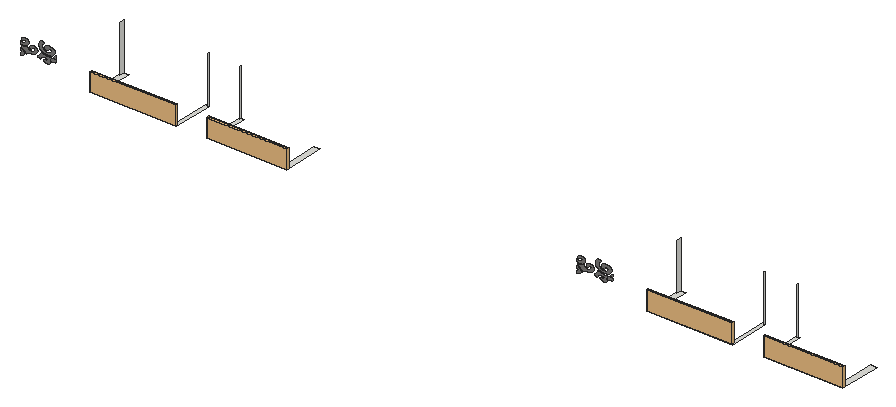
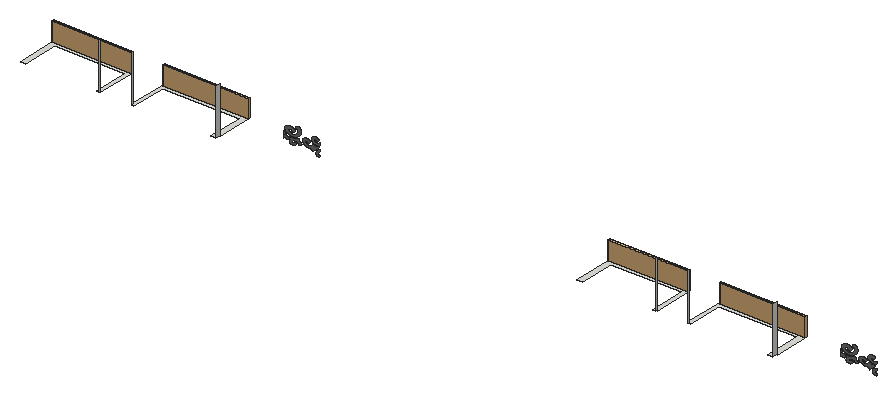
# SketchUp Ruby script. Lengths in inches.
U = 1.inch
M = Sketchup.active_model
def pt(a) = Geom::Point3d.new(a.map { |v| v * U })
def face(e, loops, mat)
  f = e.add_face(loops[0].map { |a| pt(a) })
  loops[1..].each { |l| e.add_face(l.map { |a| pt(a) }).erase! }
  f.material = f.back_material = mat if mat
  f
end
# faces: each face lists its corners as indices into pts; further lists are holes
def faces(e, pts, list, mat = nil) = list.each { |f| face(e, (f[0].is_a?(Array) ? f : [f]).map { |l| l.map { |i| pts[i] } }, mat) }
# xy, xz, yz: faces in a plane at the given z, y or x. An outline is a flat list of corners, or four numbers for a rectangle; further outlines are holes
def ring(l) = l.size == 4 ? [[l[0], l[1]], [l[2], l[1]], [l[2], l[3]], [l[0], l[3]]] : l.each_slice(2).to_a
def flat(e, list, mat, &to3) = list.each { |f| face(e, (f[0].is_a?(Array) ? f : [f]).map { |l| ring(l).map { |u, v| to3.(u, v) } }, mat) }
def xy(e, z, list, mat = nil) = flat(e, list, mat) { |x, y| [x, y, z] }
def xz(e, y, list, mat = nil) = flat(e, list, mat) { |x, z| [x, y, z] }
def yz(e, x, list, mat = nil) = flat(e, list, mat) { |y, z| [x, y, z] }
def lines(e, pts, list) = list.each { |a, b| e.add_line(pt(pts[a]), pt(pts[b])) }
# prism: a flat outline (further loops are holes) pulled along v
def prism(e, loops, v, mat = nil)
  f = face(e, loops, mat); d = Geom::Vector3d.new(v.map { |x| x * U })
  f.pushpull(f.normal.samedirection?(d) ? d.length : -d.length)
end
def box(e, o, s, mat = nil) = prism(e, [[o, [o[0] + s[0], o[1], o[2]], [o[0] + s[0], o[1] + s[1], o[2]], [o[0], o[1] + s[1], o[2]]]], [0, 0, s[2]], mat)
def at(x, y, z, deg = 0) = Geom::Transformation.translation(pt([x, y, z])) * Geom::Transformation.rotation(ORIGIN, Z_AXIS, deg.degrees)
def axes(o, x, y, z) = Geom::Transformation.new([*x, 0, *y, 0, *z, 0, *pt(o).to_a, 1])
def part(name) = M.definitions.add(name)
# library, detail: a bought-in or finely detailed component or shape, given as its bounding box
def library(name, o, s) = part(name).tap { |d| box(d.entities, o, s) }
def detail(e, o, s) = box(e.add_group.entities, o, s)
def put(e, d, t, mat = nil) = e.add_instance(d, t).tap { |i| i.material = mat if mat }
def group(e, t, mat = nil) = e.add_group.tap { |g| g.transformation = t; g.material = mat if mat }.entities
root = M.entities
M.materials.add("[0043_SaddleBrown]4").color = [124, 123, 122]
c1 = library("Glass Railing",[0,0,0],[139.5,4.76,42])
xy(root,665.9375,[[3051.13,558.125,3245.44,558.125,3245.44,647.91,3243.69,647.91,3243.69,651.03,3237.9,651.03,3237.9,570.83,3064.33,570.83,3064.33,651.03,3053.01,651.03,3053.01,640.11,3051.13,640.11],[3314.06,558.125,3493.19,558.125,3493.19,651.03,3480.11,651.03,3480.11,570.83,3322.22,570.83,3322.22,651.03,3315.93,651.03,3315.93,648.85,3314.06,648.85],[4301.76,558.125,4496.07,558.125,4496.07,647.91,4494.32,647.91,4494.32,651.03,4488.53,651.03,4488.53,570.83,4314.96,570.83,4314.96,651.03,4303.63,651.03,4303.63,640.11,4301.76,640.11],[4564.68,558.125,4743.81,558.125,4743.81,651.03,4730.74,651.03,4730.74,570.83,4572.84,570.83,4572.84,651.03,4566.56,651.03,4566.56,648.85,4564.68,648.85]])
xz(root,589.17,[[2869.93,664.9,2871.18,664.96,2872.4,665.14,2873.5625,665.43,2874.64,665.82,2875.61,666.3125,2876.44,666.89,2877.125,667.53,2877.64,668.23,2877.98,668.98,2878.13,669.74,2878.1,670.51,2877.87,671.27,2877.52,672,2877.11,672.72,2876.64,673.43,2876.1,674.125,2875.52,674.8,2874.87,675.45,2874.17,676.09,2873.42,676.7,2872.62,677.28,2871.77,677.84,2870.87,678.375,2869.93,678.88,2869.93,674.84,2871.02,674.56,2871.98,674.14,2872.78,673.61,2873.38,672.99,2873.75,672.3,2873.875,671.58,2873.75,670.86,2873.38,670.18,2872.78,669.56,2871.98,669.03,2871.02,668.61,2869.93,668.33],[4120.56,664.9,4121.81,664.96,4123.03,665.14,4124.1875,665.43,4125.26,665.82,4126.23,666.3125,4127.07,666.89,4127.75,667.53,4128.27,668.23,4128.61,668.98,4128.76,669.74,4128.72,670.51,4128.49,671.27,4128.14,672,4127.73,672.72,4127.26,673.43,4126.73,674.125,4126.14,674.8,4125.5,675.45,4124.8,676.09,4124.05,676.7,4123.24,677.28,4122.39,677.84,4121.5,678.375,4120.56,678.88,4120.56,674.84,4121.64,674.56,4122.61,674.14,4123.4,673.61,4124,672.99,4124.375,672.3,4124.5,671.58,4124.375,670.86,4124,670.18,4123.4,669.56,4122.61,669.03,4121.64,668.61,4120.56,668.33],[2929.49,668.74,2931.15,668.77,2932.76,669,2934.27,669.43,2935.6,670.04,2936.7,670.81,2937.52,671.69,2936.96,672.49,2936.51,673.32,2936.1875,674.17,2935.99,675.03,2935.91,675.91,2935.96,676.78,2936.14,677.64,2936.4375,678.5,2936.86,679.33,2937.4,680.14,2938.06,680.91,2938.82,681.65,2936.94,681.55,2935.06,681.52,2933.17,681.56,2931.29,681.66,2929.43,681.84,2927.59,682.08,2925.77,682.38,2923.98,682.76,2922.23,683.19,2920.53,683.6875,2918.88,684.25,2917.28,684.86,2917.16,683.95,2916.93,683.05,2916.59,682.16,2916.15,681.29,2915.6,680.44,2914.94,679.625,2914.19,678.84,2913.35,678.09,2912.41,677.375,2911.4,676.71,2910.3,676.1,2909.13,675.53,2909.75,675.36,2910.36,675.18,2910.97,674.99,2911.57,674.79,2912.16,674.59,2912.75,674.38,2913.33,674.16,2913.9,673.9375,2914.46,673.71,2915.02,673.47,2915.57,673.22,2916.11,672.97,2916.21,674.16,2916.74,675.32,2917.66,676.37,2918.93,677.28,2920.5,677.99,2922.27,678.48,2924.18,678.72,2926.13,678.7,2928.02,678.42,2929.77,677.89,2931.3,677.15,2932.52,676.22,2932.55,675.93,2932.57,675.64,2932.58,675.35,2932.57,675.06,2932.55,674.77,2932.51,674.48,2932.46,674.1875,2932.4,673.9,2932.32,673.61,2932.23,673.33,2932.12,673.05,2932,672.77,2931.41,672.61,2930.78,672.51,2930.13,672.47,2929.49,672.5,2928.86,672.59,2928.26,672.74,2927.7,672.95,2927.21,673.21,2926.79,673.51,2926.45,673.85,2926.21,674.22,2926.07,674.61,2925.66,674.5,2925.27,674.375,2924.89,674.24,2924.52,674.08,2924.18,673.92,2923.84,673.74,2923.53,673.55,2923.24,673.34,2922.97,673.13,2922.72,672.9,2922.5,672.67,2922.3,672.43,2922.89,671.47,2923.78,670.61,2924.9375,669.88,2926.3125,669.3125,2927.85,668.93],[4180.11,668.74,4181.77,668.77,4183.39,669,4184.89,669.43,4186.23,670.04,4187.32,670.81,4188.15,671.69,4187.58,672.49,4187.14,673.32,4186.8125,674.17,4186.61,675.03,4186.54,675.91,4186.59,676.78,4186.76,677.64,4187.0625,678.5,4187.49,679.33,4188.03,680.14,4188.68,680.91,4189.45,681.65,4187.57,681.55,4185.68,681.52,4183.8,681.56,4181.92,681.66,4180.06,681.84,4178.21,682.08,4176.39,682.38,4174.61,682.76,4172.86,683.19,4171.16,683.6875,4169.5,684.25,4167.91,684.86,4167.79,683.95,4167.56,683.05,4167.22,682.16,4166.77,681.29,4166.22,680.44,4165.57,679.625,4164.82,678.84,4163.97,678.09,4163.04,677.375,4162.02,676.71,4160.92,676.1,4159.76,675.53,4160.375,675.36,4160.99,675.18,4161.59,674.99,4162.19,674.79,4162.78,674.59,4163.37,674.38,4163.95,674.16,4164.52,673.9375,4165.09,673.71,4165.64,673.47,4166.19,673.22,4166.73,672.97,4166.84,674.16,4167.36,675.32,4168.29,676.37,4169.56,677.28,4171.12,677.99,4172.9,678.48,4174.81,678.72,4176.75,678.7,4178.65,678.42,4180.4,677.89,4181.92,677.15,4183.14,676.22,4183.18,675.93,4183.2,675.64,4183.21,675.35,4183.2,675.06,4183.18,674.77,4183.14,674.48,4183.09,674.1875,4183.03,673.9,4182.95,673.61,4182.75,673.05,4182.63,672.77,4182.03,672.61,4181.41,672.51,4180.76,672.47,4180.11,672.5,4179.48,672.59,4178.88,672.74,4178.33,672.95,4177.84,673.21,4177.42,673.51,4177.08,673.85,4176.84,674.22,4176.69,674.61,4176.29,674.5,4175.89,674.375,4175.51,674.24,4175.15,674.08,4174.8,673.92,4174.47,673.74,4174.16,673.55,4173.87,673.34,4173.6,673.13,4173.35,672.9,4173.125,672.67,4172.92,672.43,4173.51,671.47,4174.4,670.61,4175.5625,669.88,4176.9375,669.3125,4178.48,668.93],[2883.92,672.07,2884.53,672.74,2885.24,673.37,2886.0625,673.94,2886.97,674.47,2887.96,674.93,2889.02,675.33,2890.14,675.66,2891.3125,675.92,2892.52,676.11,2893.76,676.22,2895,676.25,2896.24,676.2,2898.66,676.55,2900.95,677.15,2903.02,677.98,2904.83,679.02,2906.32,680.24,2907.4375,681.61,2908.15,683.07,2908.4375,684.58,2908.29,686.1,2907.71,687.59,2906.73,688.98,2905.36,690.26,2904.23,690.96,2902.89,691.5,2901.39,691.86,2899.8,692.01,2898.2,691.96,2896.65,691.7,2895.22,691.25,2893.98,690.62,2892.98,689.85,2892.27,688.96,2891.87,688.01,2891.8125,687.02,2891.875,686.71,2891.99,686.41,2892.15,686.12,2892.36,685.84,2892.62,685.57,2892.92,685.32,2893.25,685.09,2893.63,684.89,2894.04,684.71,2894.48,684.55,2894.94,684.43,2895.41,684.33,2895.5,684.77,2895.62,685.2,2895.78,685.625,2895.99,686.04,2896.23,686.45,2896.51,686.86,2896.83,687.25,2897.18,687.625,2897.58,687.99,2898,688.34,2898.46,688.68,2898.95,689,2899.88,688.71,2900.73,688.34,2901.48,687.89,2902.11,687.37,2902.6,686.8,2902.9375,686.2,2903.125,685.57,2903.15,684.92,2903.01,684.29,2902.72,683.67,2902.27,683.09,2901.6875,682.56,2900.85,681.75,2899.78,681.0625,2898.53,680.5,2897.125,680.09,2895.62,679.85,2894.07,679.78,2892.53,679.89,2891.05,680.18,2889.68,680.62,2888.46,681.21,2887.45,681.94,2886.67,682.76,2886.45,682.98,2886.25,683.2,2886.06,683.43,2885.88,683.66,2885.71,683.9,2885.56,684.14,2885.42,684.38,2885.29,684.625,2885.17,684.87,2885.07,685.12,2884.98,685.37,2884.91,685.625,2884.22,685.06,2883.41,684.55,2882.52,684.11,2881.54,683.74,2880.49,683.45,2879.39,683.24,2878.26,683.11,2877.11,683.07,2875.97,683.125,2874.84,683.26,2873.75,683.48,2872.71,683.79,2872.92,683.52,2873.12,683.25,2873.28,682.98,2873.42,682.69,2873.54,682.4,2873.62,682.11,2873.68,681.82,2873.71,681.53,2873.72,681.23,2873.69,680.93,2873.64,680.64,2873.5625,680.35,2874.7,679.8125,2875.8,679.25,2876.86,678.65,2877.86,678.02,2878.81,677.36,2879.72,676.67,2880.5625,675.96,2881.36,675.22,2882.09,674.47,2882.76,673.6875,2883.37,672.89],
  [4134.54,672.07,4135.15,672.74,4135.87,673.37,4136.6875,673.94,4137.59,674.47,4138.58,674.93,4139.65,675.33,4140.77,675.66,4141.9375,675.92,4143.15,676.11,4144.38,676.22,4145.625,676.25,4146.87,676.2,4149.29,676.55,4151.57,677.15,4153.65,677.98,4155.46,679.02,4156.94,680.24,4158.0625,681.61,4158.77,683.07,4159.0625,684.58,4158.92,686.1,4158.34,687.59,4157.35,688.98,4155.98,690.26,4154.85,690.96,4153.51,691.5,4152.01,691.86,4150.43,692.01,4148.82,691.96,4147.27,691.7,4145.84,691.25,4144.6,690.62,4143.6,689.85,4142.89,688.96,4142.5,688.01,4142.4375,687.02,4142.5,686.71,4142.61,686.41,4142.77,686.12,4142.98,685.84,4143.24,685.57,4143.54,685.32,4143.88,685.09,4144.26,684.89,4144.66,684.71,4145.1,684.55,4145.56,684.43,4146.04,684.33,4146.12,684.77,4146.24,685.2,4146.41,685.625,4146.61,686.04,4146.85,686.45,4147.14,686.86,4147.45,687.25,4147.81,687.625,4148.2,687.99,4148.625,688.34,4149.08,688.68,4149.57,689,4150.51,688.71,4151.36,688.34,4152.11,687.89,4152.73,687.37,4153.22,686.8,4153.5625,686.2,4153.75,685.57,4153.77,684.92,4153.64,684.29,4153.34,683.67,4152.9,683.09,4152.3125,682.56,4151.47,681.75,4150.41,681.0625,4149.15,680.5,4147.75,680.09,4146.25,679.85,4144.7,679.78,4143.16,679.89,4141.68,680.18,4140.3,680.62,4139.09,681.21,4138.07,681.94,4137.29,682.76,4136.87,683.2,4136.68,683.43,4136.5,683.66,4136.18,684.14,4136.04,684.38,4135.91,684.625,4135.8,684.87,4135.7,685.12,4135.61,685.37,4135.53,685.625,4134.84,685.06,4134.04,684.55,4133.14,684.11,4132.16,683.74,4131.12,683.45,4130.02,683.24,4128.89,683.11,4127.74,683.07,4126.59,683.125,4125.46,683.26,4124.37,683.48,4123.33,683.79,4123.55,683.52,4123.74,683.25,4123.91,682.98,4124.05,682.69,4124.16,682.4,4124.25,682.11,4124.31,681.82,4124.34,681.53,4124.34,681.23,4124.32,680.93,4124.27,680.64,4124.1875,680.35,4125.33,679.8125,4126.43,679.25,4127.48,678.65,4128.49,678.02,4129.44,677.36,4130.34,676.67,4131.1875,675.96,4131.98,675.22,4132.71,674.47,4133.39,673.6875,4134,672.89],[2942.02,675.97,2942.57,675.99,2943.03,676.05,2943.48,676.14,2943.92,676.25,2944.34,676.38,2944.74,676.54,2945.12,676.72,2945.46,676.91,2945.78,677.13,2946.07,677.36,2946.32,677.61,2946.54,677.87,2946.71,678.14,2947.06,678.02,2947.4,677.9,2947.73,677.77,2948.37,677.49,2948.67,677.34,2948.97,677.18,2949.26,677.02,2949.54,676.85,2949.8125,676.67,2950.07,676.49,2950.32,676.31,2950.32,681.23,2949.35,681.5625,2948.3,681.79,2947.21,681.91,2946.1,681.93,2945.01,681.83,2943.94,681.63,2942.95,681.33,2942.04,680.9375,2941.25,680.46,2940.6,679.91,2940.09,679.3,2939.75,678.66,2939.49,678.36,2939.33,678.04,2939.28,677.71,2939.33,677.375,2939.48,677.05,2939.74,676.76,2940.07,676.5,2940.49,676.28,2940.97,676.12,2941.48,676.01],[4192.65,675.97,4193.19,675.99,4193.66,676.05,4194.11,676.14,4194.55,676.25,4194.97,676.38,4195.37,676.54,4195.74,676.72,4196.09,676.91,4196.41,677.13,4196.69,677.36,4196.95,677.61,4197.16,677.87,4197.34,678.14,4198.02,677.9,4198.35,677.77,4198.68,677.63,4198.99,677.49,4199.3,677.34,4199.6,677.18,4199.89,677.02,4200.17,676.85,4200.4375,676.67,4200.7,676.49,4200.95,676.31,4200.95,681.23,4199.97,681.5625,4198.93,681.79,4197.84,681.91,4196.73,681.93,4195.63,681.83,4194.57,681.63,4193.57,681.33,4192.67,680.9375,4191.88,680.46,4191.22,679.91,4190.71,679.3,4190.37,678.66,4190.12,678.36,4189.96,678.04,4189.9,677.71,4189.95,677.375,4190.11,677.05,4190.36,676.76,4190.7,676.5,4191.12,676.28,4191.59,676.12,4192.11,676.01],[2949.94,684.18,2950.32,684.19,2950.32,689.38,2950.04,689.01,2949.75,688.64,2949.45,688.27,2949.13,687.91,2948.8,687.55,2948.46,687.19,2948.11,686.84,2947.75,686.49,2947.37,686.15,2946.98,685.82,2946.59,685.48,2946.18,685.16,2946.45,685,2946.75,684.85,2947.06,684.71,2947.38,684.59,2947.72,684.48,2948.08,684.39,2948.4375,684.32,2948.81,684.26,2949.18,684.22,2949.5625,684.19],[4200.57,684.18,4200.95,684.19,4200.95,689.38,4200.67,689.01,4200.375,688.64,4200.07,688.27,4199.76,687.91,4199.43,687.55,4199.09,687.19,4198.37,686.49,4198,686.15,4197.61,685.82,4197.21,685.48,4196.8,685.16,4197.08,685,4197.37,684.85,4197.68,684.71,4198.01,684.59,4198.35,684.48,4198.7,684.39,4199.0625,684.32,4199.43,684.26,4199.81,684.22,4200.1875,684.19],
  [2931.82,686.15,2934.02,686.25,2936.18,686.52,2938.26,686.97,2940.22,687.6,2942.03,688.38,2943.64,689.3,2945.04,690.35,2946.1875,691.51,2947.07,692.75,2947.67,694.06,2947.98,695.4,2947.97,696.5625,2947.6875,697.72,2947.13,698.83,2946.32,699.88,2945.27,700.85,2943.99,701.71,2942.53,702.45,2940.9,703.05,2939.15,703.5,2937.3125,703.79,2935.42,703.9,2933.53,703.85,2932.06,703.66,2930.65,703.33,2929.36,702.87,2928.2,702.27,2927.22,701.58,2926.4375,700.79,2925.875,699.93,2925.55,699.03,2925.47,698.11,2925.64,697.1875,2926.04,696.3,2926.68,695.47,2927.2,695.13,2927.81,694.86,2928.51,694.68,2929.25,694.59,2930,694.6,2930.73,694.7,2931.42,694.89,2932.02,695.16,2932.53,695.5,2932.91,695.9,2933.14,696.34,2933.03,696.64,2932.97,696.95,2932.97,697.26,2933.02,697.57,2933.13,697.87,2933.29,698.16,2933.51,698.4375,2933.77,698.7,2934.09,698.94,2934.44,699.16,2934.83,699.36,2935.26,699.52,2936.27,699.43,2937.24,699.25,2938.16,698.98,2939,698.62,2939.74,698.1875,2940.37,697.69,2940.86,697.14,2941.21,696.56,2941.41,695.94,2941.46,695.3125,2941.34,694.69,2941.07,694.09,2940.33,693.08,2939.32,692.16,2938.07,691.35,2936.625,690.6875,2935.02,690.18,2933.3,689.85,2931.51,689.69,2929.7,689.72,2927.93,689.9375,2926.24,690.33,2924.6875,690.89,2923.3,691.6,2921.85,692.61,2920.63,693.73,2919.66,694.93,2918.95,696.2,2918.52,697.52,2918.375,698.87,2918.52,700.21,2918.95,701.53,2919.66,702.8,2920.63,704,2921.85,705.12,2923.3,706.125,2922.94,706.42,2922.56,706.71,2922.15,706.98,2921.73,707.24,2921.28,707.49,2920.82,707.73,2920.34,707.96,2919.85,708.17,2919.34,708.36,2918.8125,708.55,2918.27,708.71,2917.72,708.87,2916.6,707.95,2915.59,706.98,2914.7,705.98,2913.9375,704.93,2913.3,703.85,2912.8,702.75,2912.43,701.625,2912.2,700.49,2912.1,699.34,2912.15,698.19,2912.33,697.05,2912.65,695.92,2913.18,694.7,2913.91,693.52,2914.84,692.4,2915.94,691.33,2917.22,690.34,2918.65,689.4375,2920.22,688.63,2921.92,687.92,2923.73,687.32,2925.63,686.84,2927.6,686.48,2929.62,686.25],[4182.45,686.15,4184.65,686.25,4186.81,686.52,4188.89,686.97,4190.85,687.6,4192.65,688.38,4194.27,689.3,4195.66,690.35,4196.8125,691.51,4197.7,692.75,4198.3,694.06,4198.6,695.4,4198.6,696.5625,4198.3125,697.72,4197.76,698.83,4196.95,699.88,4195.89,700.85,4194.62,701.71,4193.15,702.45,4191.53,703.05,4189.77,703.5,4187.9375,703.79,4186.05,703.9,4184.15,703.85,4182.68,703.66,4181.28,703.33,4179.98,702.87,4178.83,702.27,4177.84,701.58,4177.0625,700.79,4176.5,699.93,4176.18,699.03,4176.09,698.11,4176.26,697.1875,4176.67,696.3,4177.31,695.47,4177.82,695.13,4178.44,694.86,4179.13,694.68,4179.87,694.59,4180.62,694.6,4181.36,694.7,4182.04,694.89,4182.65,695.16,4183.15,695.5,4183.53,695.9,4183.77,696.34,4183.65,696.64,4183.59,696.95,4183.59,697.26,4183.65,697.57,4183.75,697.87,4183.92,698.16,4184.13,698.4375,4184.4,698.7,4184.71,698.94,4185.07,699.16,4185.46,699.36,4185.88,699.52,4186.89,699.43,4187.87,699.25,4188.79,698.98,4189.63,698.62,4190.37,698.1875,4190.99,697.69,4191.49,697.14,4191.84,696.56,4192.04,695.94,4192.08,695.3125,4191.97,694.69,4191.7,694.09,4190.95,693.08,4189.94,692.16,4188.7,691.35,4187.25,690.6875,4185.64,690.18,4183.92,689.85,4182.14,689.69,4180.33,689.72,4178.56,689.9375,4176.87,690.33,4175.3125,690.89,4173.93,691.6,4172.48,692.61,4171.26,693.73,4170.28,694.93,4169.57,696.2,4169.15,697.52,4169,698.87,4169.15,700.21,4169.57,701.53,4170.28,702.8,4171.26,704,4172.48,705.12,4173.93,706.125,4173.57,706.42,4173.18,706.71,4172.78,706.98,4172.35,707.24,4171.91,707.49,4171.45,707.73,4170.97,707.96,4170.47,708.17,4169.96,708.36,4169.4375,708.55,4168.9,708.71,4168.35,708.87,4167.23,707.95,4166.22,706.98,4165.33,705.98,4164.5625,704.93,4163.93,703.85,4163.42,702.75,4163.05,701.625,4162.82,700.49,4162.73,699.34,4162.77,698.19,4162.96,697.05,4163.28,695.92,4163.81,694.7,4164.54,693.52,4165.46,692.4,4166.57,691.33,4167.84,690.34,4169.27,689.4375,4170.85,688.63,4172.55,687.92,4174.36,687.32,4176.26,686.84,4178.22,686.48,4180.24,686.25],[2876.93,686.97,2878,687.01,2879.07,687.11,2880.11,687.28,2881.12,687.51,2882.09,687.79,2883.79,688.47,2885.29,689.3,2886.55,690.27,2887.54,691.36,2888.24,692.52,2888.62,693.74,2888.68,694.98,2888.42,696.21,2887.84,697.4,2886.95,698.52,2885.79,699.53,2884.375,700.42,2883.4,700.93,2882.28,701.32,2881.06,701.57,2879.79,701.68,2878.5,701.64,2877.26,701.45,2876.09,701.11,2875.05,700.65,2874.17,700.08,2873.48,699.41,2873,698.68,2872.76,697.9,2872.67,697.61,2872.68,697.3,2872.78,697,2872.97,696.72,2873.25,696.47,2873.6,696.26,2874.02,696.09,2874.48,695.98,2874.96,695.92,2875.46,695.92,2875.94,695.98,2876.4,696.1,2876.67,696.3125,2876.96,696.52,2877.27,696.71,2877.59,696.89,2877.94,697.06,2878.3,697.21,2878.68,697.35,2879.07,697.48,2879.48,697.59,2879.89,697.68,2880.3125,697.76,2880.74,697.82,2881.31,697.53,2881.8,697.1875,2882.23,696.82,2882.58,696.42,2882.85,695.99,2883.03,695.55,2883.13,695.1,2883.13,694.64,2883.04,694.1875,2882.86,693.75,2882.6,693.32,2882.25,692.92,2881.52,692.31,2880.63,691.79,2879.62,691.36,2878.5,691.05,2877.3125,690.86,2876.09,690.8,2874.87,690.86,2873.68,691.05,2872.5625,691.36,2871.55,691.79,2870.66,692.31,2869.93,692.92,2869.93,688.45,2870.81,688.0625,2871.74,687.73,2872.72,687.46,2873.74,687.24,2874.79,687.09,2875.85,687],[4127.55,686.97,4128.63,687.01,4129.69,687.11,4130.74,687.28,4131.75,687.51,4132.72,687.79,4134.41,688.47,4135.91,689.3,4137.17,690.27,4138.16,691.36,4138.86,692.52,4139.24,693.74,4139.31,694.98,4139.04,696.21,4138.46,697.4,4137.58,698.52,4136.41,699.53,4135,700.42,4134.02,700.93,4132.9,701.32,4131.68,701.57,4130.41,701.68,4129.13,701.64,4127.88,701.45,4126.72,701.11,4125.67,700.65,4124.79,700.08,4124.1,699.41,4123.625,698.68,4123.39,697.9,4123.3,697.61,4123.3,697.3,4123.4,697,4123.6,696.72,4123.875,696.47,4124.23,696.26,4124.64,696.09,4125.1,695.98,4125.59,695.92,4126.08,695.92,4126.57,695.98,4127.03,696.1,4127.29,696.3125,4127.58,696.52,4127.89,696.71,4128.22,696.89,4128.57,697.06,4128.93,697.21,4129.31,697.35,4129.7,697.48,4130.1,697.59,4130.51,697.68,4130.9375,697.76,4131.37,697.82,4131.93,697.53,4132.43,697.1875,4132.86,696.82,4133.21,696.42,4133.48,695.99,4133.66,695.55,4133.75,695.1,4133.75,694.64,4133.66,694.1875,4133.49,693.75,4133.22,693.32,4132.87,692.92,4132.14,692.31,4131.26,691.79,4130.24,691.36,4129.125,691.05,4127.9375,690.86,4126.71,690.8,4125.49,690.86,4124.3,691.05,4123.1875,691.36,4122.17,691.79,4121.29,692.31,4120.56,692.92,4120.56,688.45,4121.43,688.0625,4122.36,687.73,4123.34,687.46,4124.36,687.24,4125.41,687.09,4126.48,687]],"[0043_SaddleBrown]4")
xz(root,651.03,[[3315.93,665.9375,3316.14,771.4375],[4566.56,665.9375,4566.77,771.4375]])
yz(root,3053.01,[[640.11,665.9375,651.03,771.4375]])
yz(root,3243.69,[[647.91,665.9375,651.03,771.4375]])
yz(root,3315.93,[[648.85,665.9375,651.03,771.4375]])
yz(root,4303.63,[[640.11,665.9375,651.03,771.4375]])
yz(root,4494.32,[[647.91,665.9375,651.03,771.4375]])
yz(root,4566.56,[[648.85,665.9375,651.03,771.4375]])
put(root,c1,axes([3051.13,558.125,665.9375],[1.37946,0,0],[0,1,0],[0,0,1]))
put(root,c1,axes([3314.06,558.125,665.9375],[1.28407,0,0],[0,1,0],[0,0,1]))
put(root,c1,axes([4301.76,558.125,665.9375],[1.37946,0,0],[0,1,0],[0,0,1]))
put(root,c1,axes([4564.68,558.125,665.9375],[1.28407,0,0],[0,1,0],[0,0,1]))
